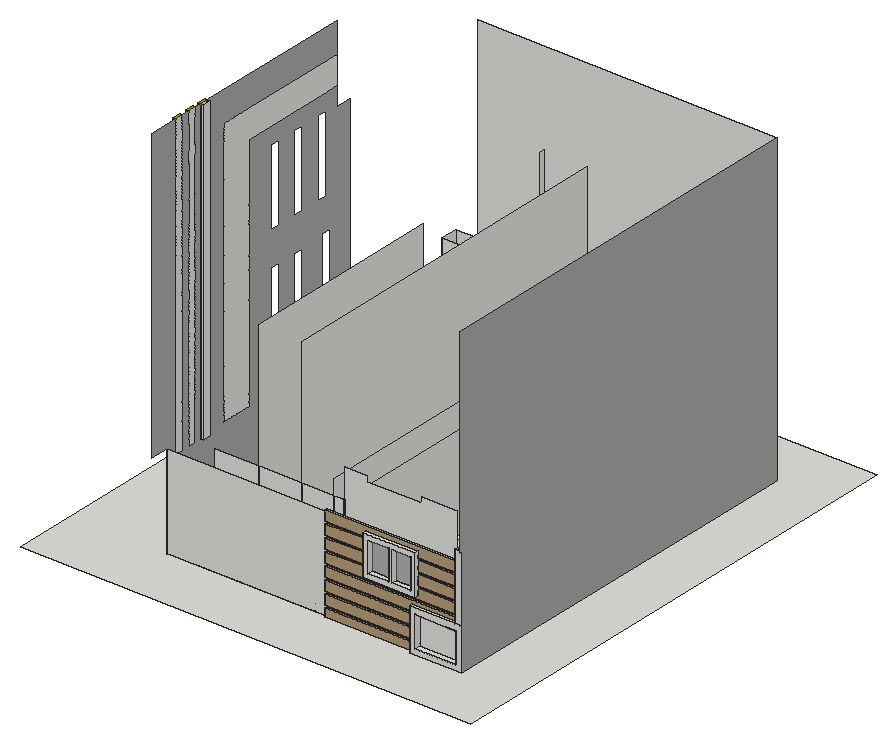
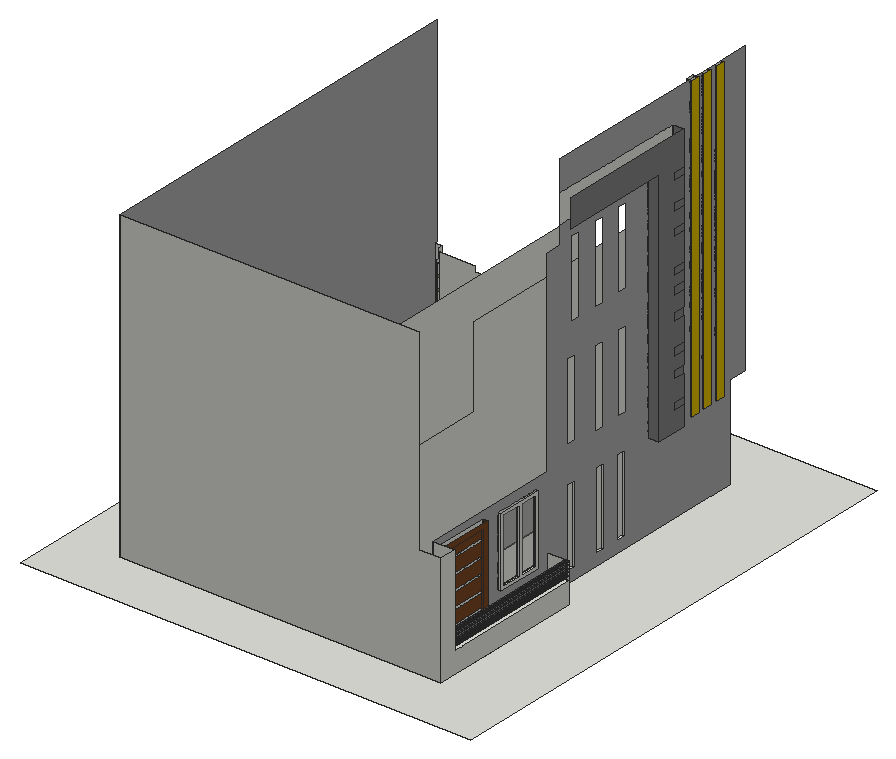
# SketchUp Ruby script. Lengths in inches.
U = 1.inch
M = Sketchup.active_model
def pt(a) = Geom::Point3d.new(a.map { |v| v * U })
def face(e, loops, mat)
  f = e.add_face(loops[0].map { |a| pt(a) })
  loops[1..].each { |l| e.add_face(l.map { |a| pt(a) }).erase! }
  f.material = f.back_material = mat if mat
  f
end
# faces: each face lists its corners as indices into pts; further lists are holes
def faces(e, pts, list, mat = nil) = list.each { |f| face(e, (f[0].is_a?(Array) ? f : [f]).map { |l| l.map { |i| pts[i] } }, mat) }
# xy, xz, yz: faces in a plane at the given z, y or x. An outline is a flat list of corners, or four numbers for a rectangle; further outlines are holes
def ring(l) = l.size == 4 ? [[l[0], l[1]], [l[2], l[1]], [l[2], l[3]], [l[0], l[3]]] : l.each_slice(2).to_a
def flat(e, list, mat, &to3) = list.each { |f| face(e, (f[0].is_a?(Array) ? f : [f]).map { |l| ring(l).map { |u, v| to3.(u, v) } }, mat) }
def xy(e, z, list, mat = nil) = flat(e, list, mat) { |x, y| [x, y, z] }
def xz(e, y, list, mat = nil) = flat(e, list, mat) { |x, z| [x, y, z] }
def yz(e, x, list, mat = nil) = flat(e, list, mat) { |y, z| [x, y, z] }
def lines(e, pts, list) = list.each { |a, b| e.add_line(pt(pts[a]), pt(pts[b])) }
# prism: a flat outline (further loops are holes) pulled along v
def prism(e, loops, v, mat = nil)
  f = face(e, loops, mat); d = Geom::Vector3d.new(v.map { |x| x * U })
  f.pushpull(f.normal.samedirection?(d) ? d.length : -d.length)
end
def box(e, o, s, mat = nil) = prism(e, [[o, [o[0] + s[0], o[1], o[2]], [o[0] + s[0], o[1] + s[1], o[2]], [o[0], o[1] + s[1], o[2]]]], [0, 0, s[2]], mat)
def at(x, y, z, deg = 0) = Geom::Transformation.translation(pt([x, y, z])) * Geom::Transformation.rotation(ORIGIN, Z_AXIS, deg.degrees)
def axes(o, x, y, z) = Geom::Transformation.new([*x, 0, *y, 0, *z, 0, *pt(o).to_a, 1])
def part(name) = M.definitions.add(name)
# library, detail: a bought-in or finely detailed component or shape, given as its bounding box
def library(name, o, s) = part(name).tap { |d| box(d.entities, o, s) }
def detail(e, o, s) = box(e.add_group.entities, o, s)
def put(e, d, t, mat = nil) = e.add_instance(d, t).tap { |i| i.material = mat if mat }
def group(e, t, mat = nil) = e.add_group.tap { |g| g.transformation = t; g.material = mat if mat }.entities
root = M.entities
M.materials.add("[0035_Tan]").color = [183, 157, 122]
M.materials.add("[0046_Gold]").color = [221, 186, 0]
M.materials.add("[0132_LightGray]").color = [169, 169, 169]
M.materials.add("[0133_Gray]").color = [128, 128, 128]
M.materials.add("[Translucent Glass Gray]").color = [128, 128, 128]
M.materials["[Translucent Glass Gray]"].alpha = 0.5
M.materials.add("[Wood Veneer 01]").color = [120, 70, 37]
xy(root,-0.75,[[106,70.06,143.81,95.5],[143.81,70.06,202.62,95.5],[202.62,70.06,269.16,95.5],[269.16,70.06,282.09,95.5],[282.09,70.06,287.5,95.5],
  [143.81,95.5,186.6,199.6],[186.6,95.5,269.16,199.6],[186.6,199.6,233.78,489.31]])
xy(root,0,[[[0,0,497.37,559.37],[378.18,64.06,378.18,68.06,282.09,68.06,282.09,70.06,138.64,70.06,138.64,199.6,202.62,199.6,202.62,489.31,186.6,489.31,186.6,95.5,106,95.5,106,322.08,82,322.08,82,498.31,436.31,498.31,436.31,64.06]],[378.18,64.06,378.18,70.06,279.43,70.06,279.43,95.5,405.67,95.5,405.67,64.06],[405.67,64.06,405.67,95.5,287.5,95.5,287.5,489.31,427.31,489.31,427.31,64.06],[427.31,64.06,436.31,489.31],[282.09,68.06,287.5,70.06],
  [287.5,68.06,378.18,70.06],[138.64,70.06,269.16,95.5],[269.16,70.06,279.43,95.5],[106,95.5,106,322.08,82,322.08,82,489.31,138.64,489.31,138.64,487.37,143.81,487.37,143.81,199.6,138.64,199.6,138.64,95.5],[138.64,95.5,143.81,199.6],
  [143.81,95.5,186.6,199.6],[186.6,95.5,202.62,199.6],[202.62,95.5,233.78,199.6],[233.78,95.5,269.16,199.6],[269.16,95.5,279.43,199.6],
  [279.43,95.5,282.09,199.6],[143.81,199.6,186.6,487.37],[143.81,199.6,186.6,487.37],[186.6,199.6,202.62,489.31],[202.62,199.6,233.78,489.31],
  [233.78,199.6,269.16,489.31],[269.16,199.6,279.43,489.31],[279.43,199.6,282.09,489.31],[138.64,487.37,143.81,489.31],[143.81,487.37,186.6,489.31],
  [82,489.31,138.64,498.31],[138.64,489.31,186.6,498.31],[186.6,489.31,208.53,498.31],[208.53,489.31,269.16,498.31],[269.16,489.31,279.43,498.31],
  [279.43,489.31,436.31,498.31]])
xy(root,6.3125,[[384.5,64.06,429.99,70.06]])
xy(root,9,[[282.09,68.06,378.18,70.06]],"[0035_Tan]")
xy(root,11.38,[[282.09,70.06,378.18,70.25]])
xy(root,11.38,[[282.09,68.06,378.18,70.06]],"[0035_Tan]")
xy(root,12.77,[[106,214.58,109,225.33],[106,243.33,109,254.08],[106,283.77,109,294.52]])
xy(root,22.875,[[282.09,70.06,288.87,70.25],[288.87,70.06,326.02,70.25],[326.02,70.06,378.18,70.25]])
xy(root,22.875,[[282.09,68.06,378.18,70.06]],"[0035_Tan]")
xy(root,24,[[82,322.08,106,322.08,106,410.8,100,410.8,100,416.8,103,416.8,103,466.49,100,466.49,100,472.49,106,472.49,106,479.49,82,479.49],[100,410.8,106,416.8],[103,416.8,106,466.49],[100,466.49,106,472.49]])
xy(root,25.26,[[282.09,68.06,378.18,70.06]],"[0035_Tan]")
xy(root,35.51,[[103,337.7,106,389.14]])
xy(root,36.75,[[282.09,68.06,378.18,70.06]],"[0035_Tan]")
xy(root,38.51,[[103,340.7,106,360.25],[103,363.42,106,386.14]])
xy(root,39.13,[[282.09,68.06,378.18,70.06]],"[0035_Tan]")
xy(root,40.125,[[384.5,64.06,429.99,70.06]])
xy(root,46.4375,[[378.18,64.06,436.31,64.06,436.31,64.12,428.8,64.12,428.8,68.06,378.18,68.06],[378.18,68.06,428.8,70.06]])
xy(root,50.625,[[282.09,68.06,428.8,70.06]],"[0035_Tan]")
xy(root,53.01,[[282.09,68.06,428.8,70.06]],"[0035_Tan]")
xy(root,56.43,[[326.64,64.06,384.7,68.06],[326.64,68.06,384.7,70.06]])
xy(root,61.75,[[331.96,64.06,355.67,70.06],[358.48,64.06,379.38,70.06]])
xy(root,64.5,[[326.02,68.06,326.64,70.06]])
xy(root,64.5,[[282.09,68.06,326.02,70.06],[384.7,68.06,428.8,70.06]],"[0035_Tan]")
xy(root,66.88,[[282.09,68.06,326.64,70.06],[384.7,68.06,428.8,70.06]],"[0035_Tan]")
xy(root,78.375,[[282.09,68.06,326.64,70.06],[384.7,68.06,428.8,70.06]],"[0035_Tan]")
xy(root,80.76,[[282.09,68.06,326.64,70.06],[384.7,68.06,428.8,70.06]],"[0035_Tan]")
xy(root,92.25,[[282.09,68.06,326.64,70.06],[384.7,68.06,428.8,70.06]],"[0035_Tan]")
xy(root,92.63,[[103,82.06,106,90.88],[103,99.88,106,108.69],[103,116.44,106,125.25],[106,116.44,109,125.25]])
xy(root,94.63,[[282.09,68.06,326.64,70.06],[384.7,68.06,428.8,70.06]],"[0035_Tan]")
xy(root,95.49,[[331.96,64.06,355.67,70.06],[358.48,64.06,379.38,70.06]])
xy(root,95.59,[[94,148.68,106,182.43]],"[0133_Gray]")
xy(root,97.71,[[106,214.58,109,225.33],[106,243.33,109,254.08],[106,283.77,109,294.52]])
xy(root,100.81,[[326.64,64.06,384.7,68.06],[326.64,68.06,384.7,70.06]])
xz(root,64.06,[[[378.18,0,436.31,46.4375],[384.5,6.3125,429.99,40.125]],[[326.64,56.43,384.7,100.81],[331.96,61.75,355.67,95.49],[358.48,61.75,379.38,95.49]]])
xz(root,64.12,[[428.8,46.4375,436.31,120]])
xz(root,68.06,[[282.09,0,378.18,9],[282.09,11.38,378.18,22.875],[282.09,25.26,378.18,36.75],[282.09,39.13,378.18,39.13,378.18,46.4375,428.8,46.4375,428.8,50.625,282.09,50.625],[282.09,53.01,428.8,53.01,428.8,64.5,384.7,64.5,384.7,56.43,326.64,56.43,326.64,64.5,282.09,64.5],
  [282.09,66.88,326.64,78.375],[384.7,66.88,428.8,78.375],[282.09,80.76,326.64,92.25],[384.7,80.76,428.8,92.25],[282.09,94.63,326.64,94.63,326.64,100.81,384.7,100.81,384.7,94.63,428.8,94.63,428.8,106.125,282.09,106.125]],"[0035_Tan]")
xz(root,70.06,[[106,-0.75,138.64,-0.75,138.64,0,282.09,0,282.09,103.1875,106,103.1875],[138.64,-0.75,143.81,0],[143.81,-0.75,186.6,0],[186.6,-0.75,202.62,0],[202.62,-0.75,208.53,0],
  [208.53,-0.75,269.16,0],[269.16,-0.75,282.09,0],[282.09,-0.75,287.5,0],[282.09,0,378.18,9],[384.5,6.3125,429.99,40.125],
  [282.09,11.38,378.18,22.875],[378.18,11.38,384.5,22.875],[282.09,25.26,378.18,36.75],[378.18,25.26,384.5,36.75],[282.09,39.13,282.09,50.625,428.8,50.625,428.8,46.4375,378.18,46.4375,378.18,39.13],
  [378.18,39.13,384.5,39.13,384.5,40.125,428.8,40.125,428.8,46.4375,378.18,46.4375],[282.09,53.01,282.09,64.5,326.64,64.5,326.64,56.43,384.7,56.43,384.7,64.5,428.8,64.5,428.8,53.01],[282.09,66.88,326.64,78.375],[384.7,66.88,428.8,78.375],[282.09,80.76,326.64,92.25],
  [384.7,80.76,428.8,92.25],[282.09,94.63,282.09,106.125,428.8,106.125,428.8,94.63,384.7,94.63,384.7,100.81,326.64,100.81,326.64,94.63]])
xz(root,70.06,[[282.09,9,378.18,11.38],[282.09,22.875,378.18,25.26],[282.09,36.75,378.18,39.13],[282.09,50.625,428.8,53.01],[282.09,64.5,326.64,66.88],
  [384.7,64.5,428.8,66.88],[282.09,78.375,326.64,80.76],[384.7,78.375,428.8,80.76],[282.09,92.25,326.64,94.63],[384.7,92.25,428.8,94.63]],"[0035_Tan]")
xz(root,70.06,[[331.96,61.75,355.67,95.49],[358.48,61.75,379.38,95.49]],"[Translucent Glass Gray]")
xz(root,70.25,[[282.09,11.38,378.18,22.875]])
xz(root,82.06,[[103,92.63,106,424.32]],"[0046_Gold]")
xz(root,90.88,[[103,92.63,106,424.32]],"[0046_Gold]")
xz(root,95.5,[[106,-0.75,143.81,0],[143.81,-0.75,186.6,0],[186.6,-0.75,202.62,0],[202.62,-0.75,269.16,0],[269.16,-0.75,282.09,0],
  [282.09,-0.75,287.5,0],[138.64,0,186.6,103.1875],[186.6,0,233.78,8.25],[233.78,0,269.16,8.25],[269.16,0,279.43,8.25],
  [279.43,0,282.09,8.25],[282.09,0,405.67,0,405.67,136.21,366.51,136.21,366.51,130.21,306.51,130.21,306.51,136.21,282.09,136.21],[186.6,8.25,233.78,103.1875],[233.78,8.25,269.16,103.1875],[269.16,8.25,279.43,103.1875],
  [279.43,8.25,282.09,103.1875]])
xz(root,99.88,[[103,92.63,106,424.32]],"[0046_Gold]")
xz(root,108.69,[[103,92.63,106,424.32]],"[0046_Gold]")
xz(root,116.44,[[106,92.63,109,424.32]])
xz(root,116.44,[[103,92.63,106,424.32]],"[0046_Gold]")
xz(root,125.25,[[106,92.63,109,424.32]])
xz(root,125.25,[[103,92.63,106,424.32]],"[0046_Gold]")
xz(root,148.68,[[94,95.59,106,95.59,106,390.53,94,390.53,94,213.9,94.81,213.9,94.81,205.625,94,205.625,94,156.87,94.68,156.87,94.68,148.59,94,148.59]],"[0133_Gray]")
xz(root,182.43,[[94,95.59,106,359.72]],"[0133_Gray]")
xz(root,199.6,[[143.81,-0.75,186.6,0],[186.6,-0.75,233.78,0],[233.78,-0.75,269.16,0]])
xz(root,214.58,[[106,12.77,109,97.71]])
xz(root,225.33,[[106,12.77,109,97.71]])
xz(root,243.33,[[106,12.77,109,97.71]])
xz(root,254.08,[[106,12.77,109,97.71]])
xz(root,283.77,[[106,12.77,109,97.71]])
xz(root,294.52,[[106,12.77,109,97.71]])
xz(root,322.08,[[82,0,106,24],[84.5,26.12,84.86,26.17,85.1875,26.3,85.47,26.52,85.69,26.81,85.83,27.14,85.875,27.49,85.83,27.85,85.69,28.18,85.47,28.47,85.1875,28.69,84.86,28.82,84.5,28.87,84.14,28.82,83.8125,28.69,83.53,28.47,83.31,28.18,83.17,27.85,83.125,27.49,83.17,27.14,83.31,26.81,83.53,26.52,83.8125,26.3,84.14,26.17],[84.5,30.06,84.86,30.1,85.1875,30.24,85.47,30.46,85.69,30.74,85.83,31.08,85.875,31.43,85.83,31.79,85.69,32.12,85.47,32.4,85.1875,32.62,84.86,32.76,84.5,32.81,84.14,32.76,83.8125,32.62,83.53,32.4,83.31,32.12,83.17,31.79,83.125,31.43,83.17,31.08,83.31,30.74,83.53,30.46,83.8125,30.24,84.14,30.1],[84.5,33.49,84.86,33.54,85.1875,33.68,85.47,33.9,85.69,34.18,85.83,34.51,85.875,34.87,85.83,35.23,85.69,35.56,85.47,35.84,85.1875,36.06,84.86,36.2,84.5,36.24,84.14,36.2,83.8125,36.06,83.53,35.84,83.31,35.56,83.17,35.23,83.125,34.87,83.17,34.51,83.31,34.18,83.53,33.9,83.8125,33.68,84.14,33.54],[84.5,37.31,84.86,37.35,85.1875,37.49,85.47,37.71,85.69,37.99,85.83,38.33,85.875,38.68,85.83,39.04,85.69,39.37,85.47,39.65,85.1875,39.87,84.86,40.01,84.5,40.06,84.14,40.01,83.8125,39.87,83.53,39.65,83.31,39.37,83.17,39.04,83.125,38.68,83.17,38.33,83.31,37.99,83.53,37.71,83.8125,37.49,84.14,37.35],
  [84.5,40.81,84.86,40.85,85.1875,40.99,85.47,41.21,85.69,41.49,85.83,41.83,85.875,42.18,85.83,42.54,85.69,42.87,85.47,43.15,85.1875,43.37,84.86,43.51,84.5,43.56,84.14,43.51,83.8125,43.37,83.53,43.15,83.31,42.87,83.17,42.54,83.125,42.18,83.17,41.83,83.31,41.49,83.53,41.21,83.8125,40.99,84.14,40.85]])
xz(root,337.7,[[103,35.51,106,112.39]])
xz(root,340.7,[[103,38.51,106,109.39]])
xz(root,360.25,[[103,38.51,106,109.39]])
xz(root,363.42,[[103,38.51,106,109.39]])
xz(root,386.14,[[103,38.51,106,109.39]])
xz(root,389.14,[[103,35.51,106,112.39]])
xz(root,410.8,[[100,24,106,116.0625]],"[Wood Veneer 01]")
xz(root,416.8,[[100,24,103,110.0625]],"[Wood Veneer 01]")
xz(root,466.49,[[100,24,103,110.0625]],"[Wood Veneer 01]")
xz(root,472.49,[[100,24,106,116.0625]],"[Wood Veneer 01]")
xz(root,479.49,[[[82,24,106,123.47],[84.5,33.49,84.14,33.54,83.8125,33.68,83.53,33.9,83.31,34.18,83.17,34.51,83.125,34.87,83.17,35.23,83.31,35.56,83.53,35.84,83.8125,36.06,84.14,36.2,84.5,36.24,84.86,36.2,85.1875,36.06,85.47,35.84,85.69,35.56,85.83,35.23,85.875,34.87,85.83,34.51,85.69,34.18,85.47,33.9,85.1875,33.68,84.86,33.54],[84.5,37.31,84.14,37.35,83.8125,37.49,83.53,37.71,83.31,37.99,83.17,38.33,83.125,38.68,83.17,39.04,83.31,39.37,83.53,39.65,83.8125,39.87,84.14,40.01,84.5,40.06,84.86,40.01,85.1875,39.87,85.47,39.65,85.69,39.37,85.83,39.04,85.875,38.68,85.83,38.33,85.69,37.99,85.47,37.71,85.1875,37.49,84.86,37.35],[84.5,40.81,84.14,40.85,83.8125,40.99,83.53,41.21,83.31,41.49,83.17,41.83,83.125,42.18,83.17,42.54,83.31,42.87,83.53,43.15,83.8125,43.37,84.14,43.51,84.5,43.56,84.86,43.51,85.1875,43.37,85.47,43.15,85.69,42.87,85.83,42.54,85.875,42.18,85.83,41.83,85.69,41.49,85.47,41.21,85.1875,40.99,84.86,40.85],[84.5,30.06,84.14,30.1,83.8125,30.24,83.53,30.46,83.31,30.74,83.17,31.08,83.125,31.43,83.17,31.79,83.31,32.12,83.53,32.4,83.8125,32.62,84.14,32.76,84.5,32.81,84.86,32.76,85.1875,32.62,85.47,32.4,85.69,32.12,85.83,31.79,85.875,31.43,85.83,31.08,85.69,30.74,85.47,30.46,85.1875,30.24,84.86,30.1],[84.5,26.12,84.14,26.17,83.8125,26.3,83.53,26.52,83.31,26.81,83.17,27.14,83.125,27.49,83.17,27.85,83.31,28.18,83.53,28.47,83.8125,28.69,84.14,28.82,84.5,28.87,84.86,28.82,85.1875,28.69,85.47,28.47,85.69,28.18,85.83,27.85,85.875,27.49,85.83,27.14,85.69,26.81,85.47,26.52,85.1875,26.3,84.86,26.17]]])
xz(root,487.37,[[138.64,0,186.6,120]])
xz(root,489.31,[[186.6,-0.75,208.53,0],[208.53,-0.75,233.78,0],[138.64,0,143.81,103.1875],[143.81,0,186.6,103.1875],[186.6,0,202.62,103.1875],
  [202.62,0,208.53,103.1875],[208.53,0,233.78,103.1875],[233.78,0,269.16,103.1875],[269.16,0,279.43,103.1875],[279.43,0,282.09,103.1875],
  [282.09,0,287.5,120],[287.5,0,427.31,120]])
xz(root,498.31,[[82,0,82,123.47,106,123.47,106,339,436.31,339,436.31,0]])
yz(root,82,[[322.08,0,322.08,24,479.49,24,479.49,123.47,498.31,123.47,498.31,0]])
yz(root,94,[[148.68,95.59,148.68,117.15,162.08,117.15,162.08,125.43,148.68,125.43,148.68,148.59,162.08,148.59,162.08,156.87,148.68,156.87,148.68,171.09,162.08,171.09,162.08,179.37,148.68,179.37,148.68,205.625,162.08,205.625,162.08,213.9,148.68,213.9,148.68,231.46,162.08,231.46,162.08,239.74,148.68,239.74,148.68,250.96,162.08,250.96,162.08,259.24,148.68,259.24,148.68,289.0625,162.08,289.0625,162.08,297.34,148.68,297.34,148.68,314.34,162.08,314.34,162.08,322.62,148.68,322.62,148.68,344.71,162.08,344.71,162.08,352.99,148.68,352.99,148.68,390.53,303.56,390.53,303.56,359.72,182.43,359.72,182.43,95.59]],"[0133_Gray]")
yz(root,100,[[410.8,24,410.8,116.0625,472.49,116.0625,472.49,24,466.49,24,466.49,110.0625,416.8,110.0625,416.8,24]],"[Wood Veneer 01]")
yz(root,103,[[416.8,24,456.01,28.48],[456.01,24,456.01,28.48,416.8,28.48,416.8,31.14,456.01,31.14,456.01,45.48,416.8,45.48,416.8,48.14,456.01,48.14,456.01,62.48,416.8,62.48,416.8,65.14,456.01,65.14,456.01,79.48,416.8,79.48,416.8,82.14,456.01,82.14,456.01,96.48,416.8,96.48,416.8,99.14,456.01,99.14,456.01,110.0625,458.36,110.0625,458.36,99.14,466.49,99.14,466.49,96.48,458.36,96.48,458.36,82.14,466.49,82.14,466.49,79.48,458.36,79.48,458.36,65.14,466.49,65.14,466.49,62.48,458.36,62.48,458.36,48.14,466.49,48.14,466.49,45.48,458.36,45.48,458.36,31.14,466.49,31.14,466.49,28.48,458.36,28.48,458.36,24],[458.36,24,466.49,28.48],[[337.7,35.51,389.14,112.39],[363.42,38.51,386.14,109.39],[340.7,38.51,360.25,109.39]]])
yz(root,103,[[82.06,92.63,90.88,424.32],[99.88,92.63,108.69,424.32],[116.44,92.63,125.25,424.32]],"[0046_Gold]")
yz(root,103,[[416.8,31.14,456.01,45.48],[458.36,31.14,466.49,45.48],[416.8,48.14,456.01,62.48],[458.36,48.14,466.49,62.48],[416.8,65.14,456.01,79.48],
  [458.36,65.14,466.49,79.48],[416.8,82.14,456.01,96.48],[458.36,82.14,466.49,96.48],[416.8,99.14,456.01,110.0625],[458.36,99.14,466.49,110.0625]],"[Wood Veneer 01]")
yz(root,106,[[410.8,18,472.49,24],[[337.7,35.51,389.14,112.39],[363.42,38.51,386.14,109.39],[340.7,38.51,360.25,109.39]],[82.06,92.63,90.88,424.32],[99.88,92.63,108.69,424.32],[116.44,92.63,125.25,424.32],
  [148.68,95.59,182.43,95.59,182.43,359.72,303.56,359.72,303.56,390.53,148.68,390.53]])
yz(root,106,[[[70.06,-0.75,70.06,103.1875,49.06,103.1875,49.06,424.32,82.06,424.32,82.06,92.63,90.88,92.63,90.88,424.32,99.88,424.32,99.88,92.63,108.69,92.63,108.69,424.32,116.44,424.32,116.44,92.63,125.25,92.63,125.25,424.32,303.56,424.32,303.56,390.53,148.68,390.53,148.68,95.59,182.43,95.59,182.43,359.72,303.56,359.72,303.56,339,322.08,339,322.08,123.47,479.49,123.47,479.49,24,472.49,24,472.49,116.0625,410.8,116.0625,410.8,24,322.08,24,322.08,0,95.5,0,95.5,-0.75],[337.7,35.51,389.14,112.39],[214.58,12.77,225.33,97.71],[243.33,12.77,254.08,97.71],[283.77,12.77,294.52,97.71],[283.77,137.52,294.52,222.46],[245.52,133.96,256.27,218.9],[212.89,134.96,223.64,219.9],[212.89,256.71,223.64,341.65],[244.77,256.71,255.52,341.65],[278.27,256.71,289.02,341.65]]],"[0132_LightGray]")
yz(root,106,[[340.7,38.51,360.25,109.39],[363.42,38.51,386.14,109.39]],"[Translucent Glass Gray]")
yz(root,109,[[214.58,12.77,225.33,97.71],[243.33,12.77,254.08,97.71],[283.77,12.77,294.52,97.71],[116.44,92.63,125.25,424.32]])
yz(root,138.64,[[487.37,0,489.31,120]])
yz(root,143.81,[[95.5,-0.75,199.6,0]])
yz(root,186.6,[[95.5,-0.75,199.6,0],[199.6,-0.75,487.37,0],[487.37,-0.75,489.31,0],[95.5,0,487.37,0,487.37,120,489.31,120,489.31,243,483.47,243,483.47,154.22,322.08,154.22,322.08,243,95.5,243],[487.37,0,489.31,120]])
yz(root,233.78,[[199.6,-0.75,489.31,0],[95.5,0,489.31,242.875]])
yz(root,269.16,[[70.06,-0.75,95.5,0],[95.5,-0.75,199.6,0],[95.5,0,489.31,120]])
yz(root,282.09,[[95.5,0,489.31,103.1875],[70.06,11.38,70.25,22.875]])
yz(root,282.09,[[68.06,0,70.06,9],[68.06,11.38,70.06,22.875],[68.06,25.26,70.06,36.75],[68.06,39.13,70.06,50.625],[68.06,53.01,70.06,64.5],
  [68.06,66.88,70.06,78.375],[68.06,80.76,70.06,92.25],[68.06,94.63,70.06,103.1875]],"[0035_Tan]")
yz(root,326.64,[[64.06,56.43,64.06,100.81,68.06,100.81,68.06,94.63,70.06,94.63,70.06,92.25,68.06,92.25,68.06,80.76,70.06,80.76,70.06,78.375,68.06,78.375,68.06,66.88,70.06,66.88,70.06,64.5,68.06,64.5,68.06,56.43],[68.06,56.43,70.06,64.5],[68.06,66.88,70.06,78.375],[68.06,80.76,70.06,92.25],[68.06,94.63,70.06,100.81]])
yz(root,331.96,[[64.06,61.75,70.06,95.49]])
yz(root,355.67,[[64.06,61.75,70.06,95.49]])
yz(root,358.48,[[64.06,61.75,70.06,95.49]])
yz(root,378.18,[[64.06,0,64.06,46.4375,68.06,46.4375,68.06,39.13,70.06,39.13,70.06,36.75,68.06,36.75,68.06,25.26,70.06,25.26,70.06,22.875,68.06,22.875,68.06,11.38,70.06,11.38,70.06,9,68.06,9,68.06,0],[68.06,0,70.06,9],[68.06,11.38,70.06,22.875],[70.06,11.38,70.25,22.875],[68.06,25.26,70.06,36.75],
  [68.06,39.13,70.06,46.4375]])
yz(root,379.38,[[64.06,61.75,70.06,95.49]])
yz(root,384.5,[[64.06,6.3125,70.06,40.125]])
yz(root,384.7,[[64.06,56.43,68.06,56.43,68.06,64.5,70.06,64.5,70.06,66.88,68.06,66.88,68.06,78.375,70.06,78.375,70.06,80.76,68.06,80.76,68.06,92.25,70.06,92.25,70.06,94.63,68.06,94.63,68.06,100.81,64.06,100.81],[68.06,56.43,70.06,64.5],[68.06,66.88,70.06,78.375],[68.06,80.76,70.06,92.25],[68.06,94.63,70.06,100.81]])
yz(root,428.8,[[64.12,46.4375,64.12,120,68.06,120,68.06,108.51,70.06,108.51,70.06,106.125,68.06,106.125,68.06,94.63,70.06,94.63,70.06,92.25,68.06,92.25,68.06,80.76,70.06,80.76,70.06,78.375,68.06,78.375,68.06,66.88,70.06,66.88,70.06,64.5,68.06,64.5,68.06,53.01,70.06,53.01,70.06,50.625,68.06,50.625,68.06,46.4375],[68.06,46.4375,70.06,50.625],[68.06,53.01,70.06,64.5],[68.06,66.88,70.06,78.375],[68.06,80.76,70.06,92.25],
  [68.06,94.63,70.06,106.125]])
yz(root,429.99,[[64.06,6.3125,70.06,40.125]])
yz(root,436.31,[[64.06,0,498.31,0,498.31,339,61.06,339,61.06,120,64.12,120,64.12,46.4375,64.06,46.4375]],"[0132_LightGray]")
p = [[82,322.08,24],[106,321.98,24],[106,321.98,43.3125],[82,322.08,43.3125],[84.14,479.49,26.17],[84.5,479.49,26.12],
  [84.5,322.08,26.12],[84.14,322.08,26.17],[84.86,479.49,26.17],[84.86,322.08,26.17],[83.8125,479.49,26.3],[83.8125,322.08,26.3],
  [85.1875,479.49,26.3],[85.1875,322.08,26.3],[83.53,479.49,26.52],[83.53,322.08,26.52],[85.47,479.49,26.52],[85.47,322.08,26.52],
  [83.31,479.49,26.81],[83.31,322.08,26.81],[85.69,479.49,26.81],[85.69,322.08,26.81],[83.17,479.49,27.14],[83.17,322.08,27.14],
  [85.83,479.49,27.14],[85.83,322.08,27.14],[83.125,479.49,27.49],[83.125,322.08,27.49],[85.875,479.49,27.49],[85.875,322.08,27.49],
  [83.17,479.49,27.85],[83.17,322.08,27.85],[85.83,479.49,27.85],[85.83,322.08,27.85],[83.31,479.49,28.18],[83.31,322.08,28.18],
  [85.69,479.49,28.18],[85.69,322.08,28.18],[83.53,479.49,28.47],[83.53,322.08,28.47],[85.47,479.49,28.47],[85.47,322.08,28.47],
  [83.8125,479.49,28.69],[83.8125,322.08,28.69],[85.1875,479.49,28.69],[85.1875,322.08,28.69],[84.14,479.49,28.82],[84.14,322.08,28.82],
  [84.86,479.49,28.82],[84.86,322.08,28.82],[84.5,479.49,28.87],[84.5,322.08,28.87],[83.8125,479.49,30.24],[84.14,479.49,30.1],
  [84.14,322.08,30.1],[83.8125,322.08,30.24],[84.5,479.49,30.06],[84.5,322.08,30.06],[84.86,479.49,30.1],[84.86,322.08,30.1],
  [85.1875,479.49,30.24],[85.1875,322.08,30.24],[83.53,479.49,30.46],[83.53,322.08,30.46],[85.47,479.49,30.46],[85.47,322.08,30.46],
  [83.31,479.49,30.74],[83.31,322.08,30.74],[85.69,479.49,30.74],[85.69,322.08,30.74],[83.17,479.49,31.08],[83.17,322.08,31.08],
  [85.83,479.49,31.08],[85.83,322.08,31.08],[83.125,479.49,31.43],[83.125,322.08,31.43],[85.875,479.49,31.43],[85.875,322.08,31.43],
  [83.17,479.49,31.79],[83.17,322.08,31.79],[85.83,479.49,31.79],[85.83,322.08,31.79],[83.31,479.49,32.12],[83.31,322.08,32.12],
  [85.69,479.49,32.12],[85.69,322.08,32.12],[83.53,479.49,32.4],[83.53,322.08,32.4],[85.47,479.49,32.4],[85.47,322.08,32.4],
  [83.8125,479.49,32.62],[83.8125,322.08,32.62],[85.1875,479.49,32.62],[85.1875,322.08,32.62],[84.14,479.49,32.76],[84.14,322.08,32.76],
  [84.86,479.49,32.76],[84.86,322.08,32.76],[84.5,479.49,32.81],[84.5,322.08,32.81],[83.8125,479.49,33.68],[84.14,479.49,33.54],
  [84.14,322.08,33.54],[83.8125,322.08,33.68],[84.5,479.49,33.49],[84.5,322.08,33.49],[84.86,479.49,33.54],[84.86,322.08,33.54],
  [85.1875,479.49,33.68],[85.1875,322.08,33.68],[83.53,479.49,33.9],[83.53,322.08,33.9],[85.47,479.49,33.9],[85.47,322.08,33.9],
  [83.31,479.49,34.18],[83.31,322.08,34.18],[85.69,479.49,34.18],[85.69,322.08,34.18],[83.17,479.49,34.51],[83.17,322.08,34.51],
  [85.83,479.49,34.51],[85.83,322.08,34.51],[83.125,479.49,34.87],[83.125,322.08,34.87],[85.875,479.49,34.87],[85.875,322.08,34.87],
  [83.17,479.49,35.23],[83.17,322.08,35.23],[85.83,479.49,35.23],[85.83,322.08,35.23],[83.31,479.49,35.56],[83.31,322.08,35.56],
  [85.69,479.49,35.56],[85.69,322.08,35.56],[83.53,479.49,35.84],[83.53,322.08,35.84],[85.47,479.49,35.84],[85.47,322.08,35.84],
  [83.8125,479.49,36.06],[83.8125,322.08,36.06],[85.1875,479.49,36.06],[85.1875,322.08,36.06],[84.14,479.49,36.2],[84.14,322.08,36.2],
  [84.86,479.49,36.2],[84.86,322.08,36.2],[84.5,479.49,36.24],[84.5,322.08,36.24],[84.14,479.49,37.35],[84.5,479.49,37.31],
  [84.5,322.08,37.31],[84.14,322.08,37.35],[84.86,479.49,37.35],[84.86,322.08,37.35],[83.8125,479.49,37.49],[83.8125,322.08,37.49],
  [85.1875,479.49,37.49],[85.1875,322.08,37.49],[83.53,479.49,37.71],[83.53,322.08,37.71],[85.47,479.49,37.71],[85.47,322.08,37.71],
  [83.31,479.49,37.99],[83.31,322.08,37.99],[85.69,479.49,37.99],[85.69,322.08,37.99],[83.17,479.49,38.33],[83.17,322.08,38.33],
  [85.83,479.49,38.33],[85.83,322.08,38.33],[83.125,479.49,38.68],[83.125,322.08,38.68],[85.875,479.49,38.68],[85.875,322.08,38.68],
  [83.17,479.49,39.04],[83.17,322.08,39.04],[85.83,479.49,39.04],[85.83,322.08,39.04],[83.31,479.49,39.37],[83.31,322.08,39.37],
  [85.69,479.49,39.37],[85.69,322.08,39.37],[83.53,479.49,39.65],[83.53,322.08,39.65],[85.47,479.49,39.65],[85.47,322.08,39.65],
  [83.8125,479.49,39.87],[83.8125,322.08,39.87],[85.1875,479.49,39.87],[85.1875,322.08,39.87],[84.14,479.49,40.01],[84.14,322.08,40.01],
  [84.86,479.49,40.01],[84.86,322.08,40.01],[84.5,479.49,40.06],[84.5,322.08,40.06],[84.14,479.49,40.85],[84.5,479.49,40.81],
  [84.5,322.08,40.81],[84.14,322.08,40.85],[84.86,479.49,40.85],[84.86,322.08,40.85],[83.8125,479.49,40.99],[83.8125,322.08,40.99],
  [85.1875,479.49,40.99],[85.1875,322.08,40.99],[83.53,479.49,41.21],[83.53,322.08,41.21],[85.47,479.49,41.21],[85.47,322.08,41.21],
  [83.31,479.49,41.49],[83.31,322.08,41.49],[85.69,479.49,41.49],[85.69,322.08,41.49],[83.17,479.49,41.83],[83.17,322.08,41.83],
  [85.83,479.49,41.83],[85.83,322.08,41.83],[83.125,479.49,42.18],[83.125,322.08,42.18],[85.875,479.49,42.18],[85.875,322.08,42.18],
  [83.17,479.49,42.54],[83.17,322.08,42.54],[85.83,479.49,42.54],[85.83,322.08,42.54],[83.31,479.49,42.87],[83.31,322.08,42.87],
  [85.69,479.49,42.87],[85.69,322.08,42.87],[83.53,479.49,43.15],[83.53,322.08,43.15],[85.47,479.49,43.15],[85.47,322.08,43.15],
  [83.8125,479.49,43.37],[83.8125,322.08,43.37],[85.1875,479.49,43.37],[85.1875,322.08,43.37],[84.14,479.49,43.51],[84.14,322.08,43.51],
  [84.86,479.49,43.51],[84.86,322.08,43.51],[84.5,479.49,43.56],[84.5,322.08,43.56],[138.64,199.6,0],[138.64,199.6,120],
  [269.16,70.06,8.25],[269.16,95.5,8.25],[282.09,70.06,-2.49],[282.09,70.06,-0.75],[428.8,70.06,-2.49],[428.8,70.06,6.3125],
  [378.18,70.06,9],[384.5,70.06,9],[282.09,70.06,-4.875],[288.87,70.06,-4.875],[427.31,70.06,-4.875],[427.68,70.06,-4.875]]
faces(root,p,[[0,1,2,3]])
faces(root,p,[[4,5,6,7],[5,8,9,6],[10,4,7,11],[8,12,13,9],[14,10,11,15],[12,16,17,13],[18,14,15,19],[16,20,21,17],
  [22,18,19,23],[20,24,25,21],[26,22,23,27],[24,28,29,25],[30,26,27,31],[28,32,33,29],[34,30,31,35],[32,36,37,33],
  [38,34,35,39],[36,40,41,37],[42,38,39,43],[40,44,45,41],[46,42,43,47],[44,48,49,45],[50,46,47,51],[48,50,51,49],
  [52,53,54,55],[53,56,57,54],[56,58,59,57],[58,60,61,59],[62,52,55,63],[60,64,65,61],[66,62,63,67],[64,68,69,65],
  [70,66,67,71],[68,72,73,69],[74,70,71,75],[72,76,77,73],[78,74,75,79],[76,80,81,77],[82,78,79,83],[80,84,85,81],
  [86,82,83,87],[84,88,89,85],[90,86,87,91],[88,92,93,89],[94,90,91,95],[92,96,97,93],[98,94,95,99],[96,98,99,97],
  [100,101,102,103],[101,104,105,102],[104,106,107,105],[106,108,109,107],[110,100,103,111],[108,112,113,109],[114,110,111,115],[112,116,117,113],
  [118,114,115,119],[116,120,121,117],[122,118,119,123],[120,124,125,121],[126,122,123,127],[124,128,129,125],[130,126,127,131],[128,132,133,129],
  [134,130,131,135],[132,136,137,133],[138,134,135,139],[136,140,141,137],[142,138,139,143],[140,144,145,141],[146,142,143,147],[144,146,147,145],
  [148,149,150,151],[149,152,153,150],[154,148,151,155],[152,156,157,153],[158,154,155,159],[156,160,161,157],[162,158,159,163],[160,164,165,161],
  [166,162,163,167],[164,168,169,165],[170,166,167,171],[168,172,173,169],[174,170,171,175],[172,176,177,173],[178,174,175,179],[176,180,181,177],
  [182,178,179,183],[180,184,185,181],[186,182,183,187],[184,188,189,185],[190,186,187,191],[188,192,193,189],[194,190,191,195],[192,194,195,193],
  [196,197,198,199],[197,200,201,198],[202,196,199,203],[200,204,205,201],[206,202,203,207],[204,208,209,205],[210,206,207,211],[208,212,213,209],
  [214,210,211,215],[212,216,217,213],[218,214,215,219],[216,220,221,217],[222,218,219,223],[220,224,225,221],[226,222,223,227],[224,228,229,225],
  [230,226,227,231],[228,232,233,229],[234,230,231,235],[232,236,237,233],[238,234,235,239],[236,240,241,237],[242,238,239,243],[240,242,243,241]],"[0133_Gray]")
lines(root,p,[[244,245],[246,247],[248,249],[250,251],[252,253],[254,255],[256,257]])
